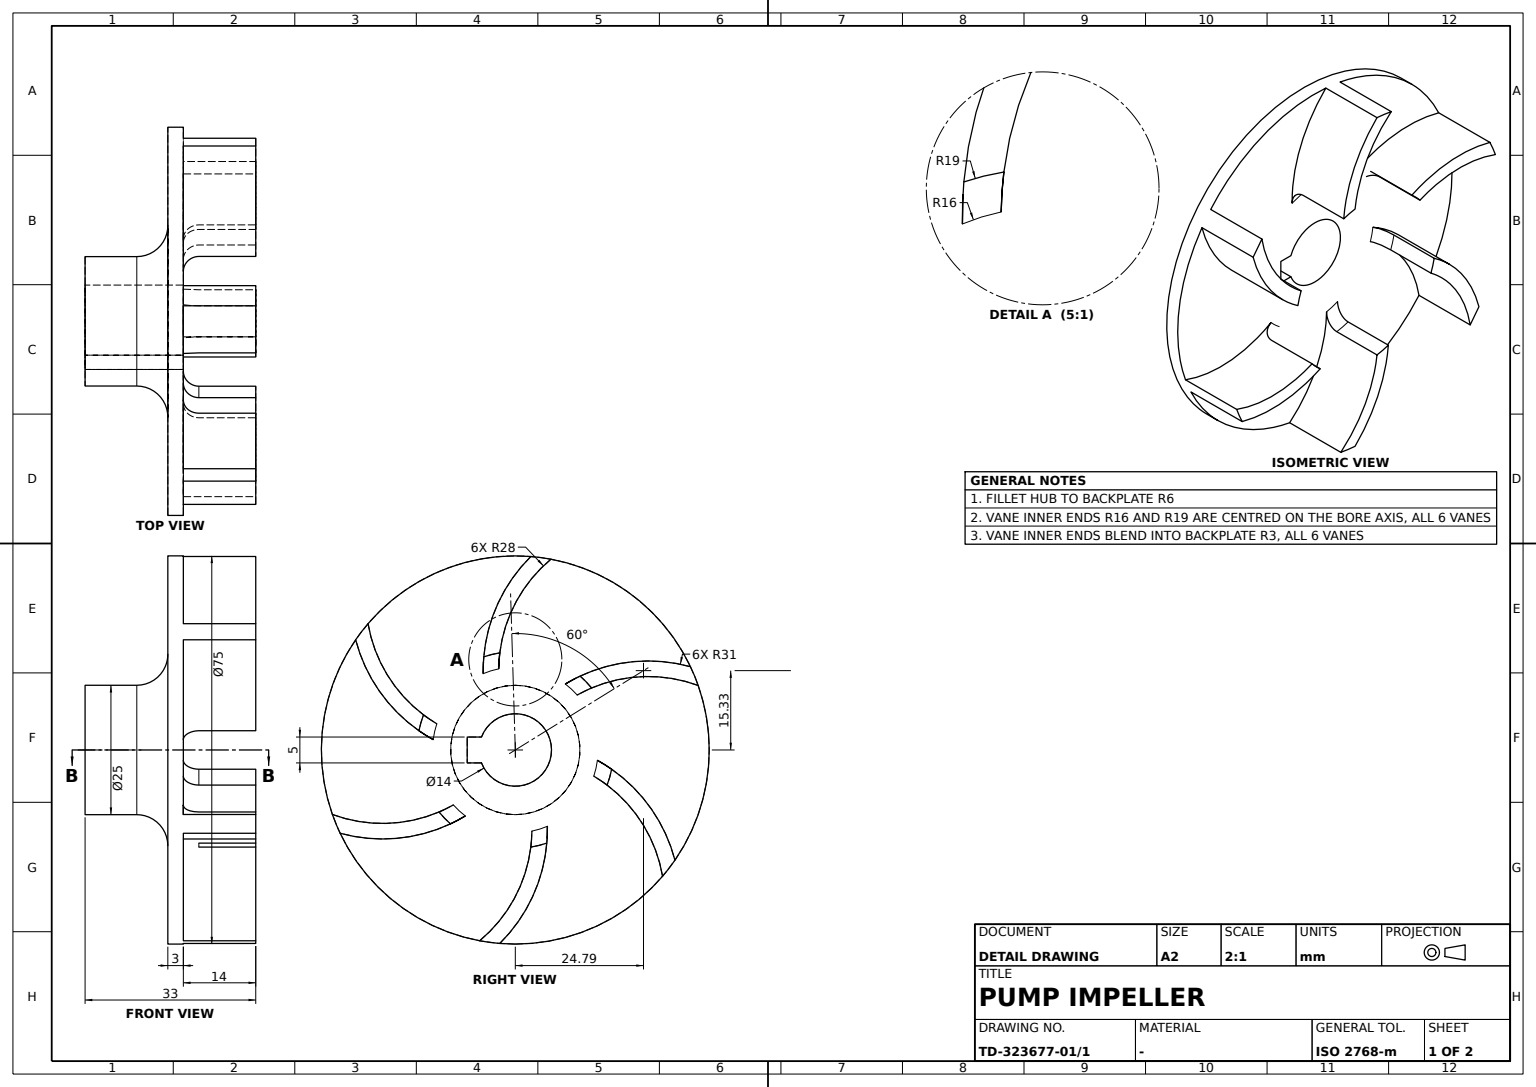
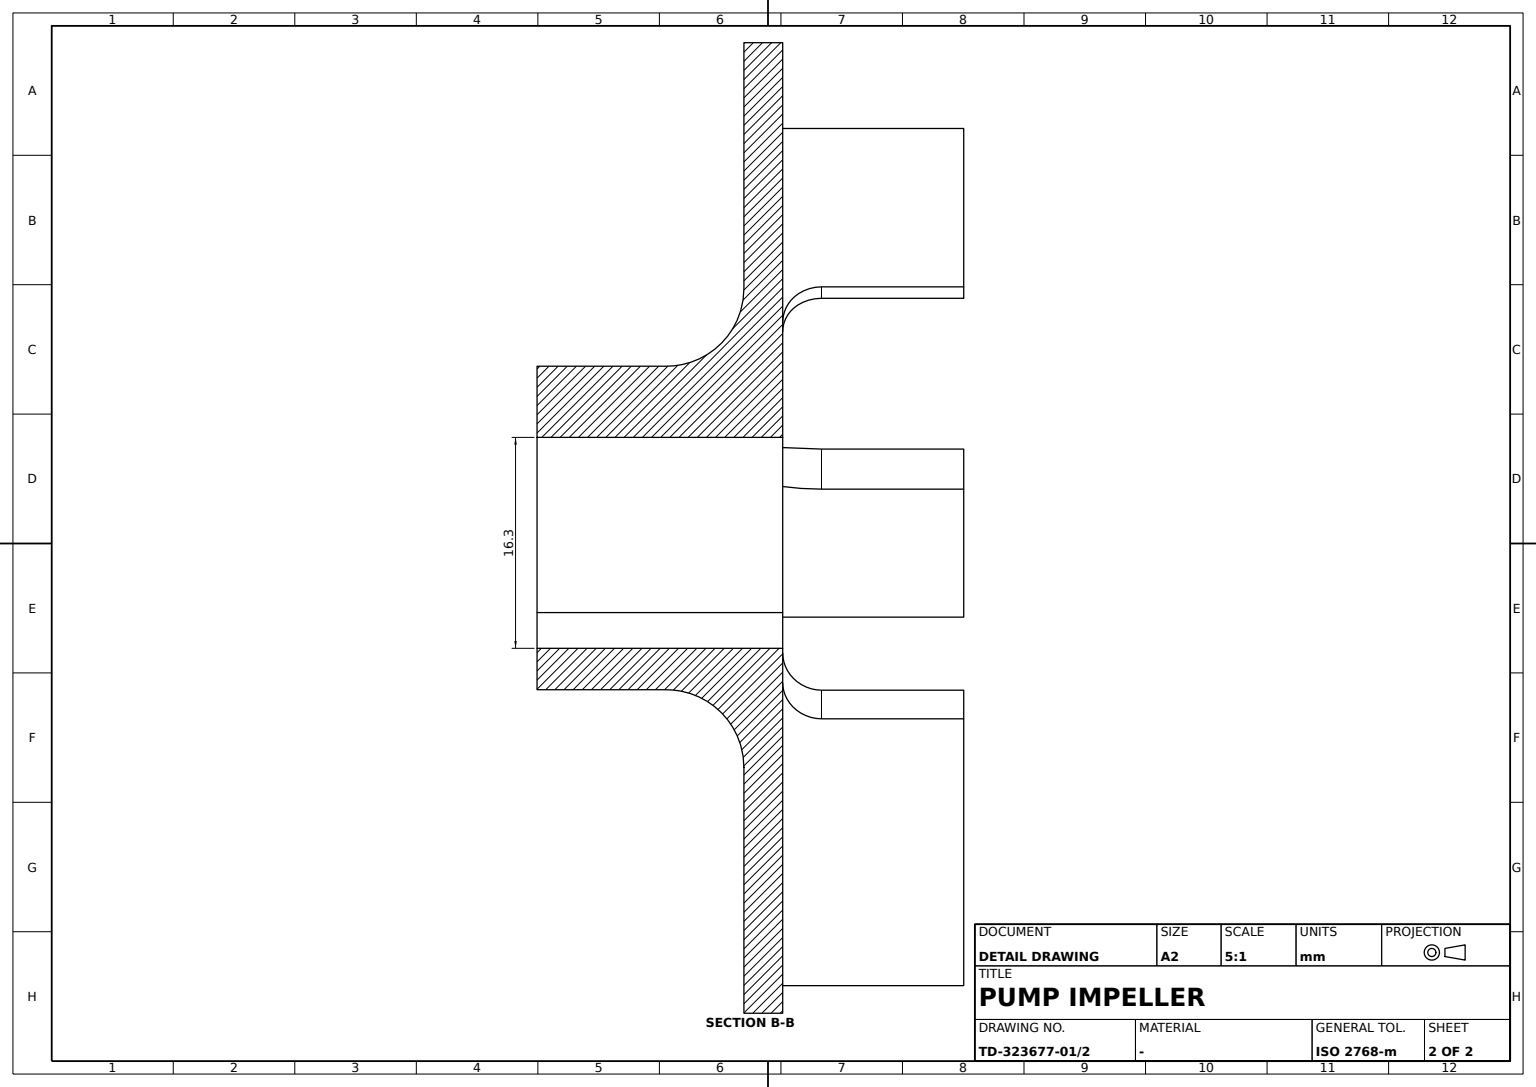
ISO-10303-21;
HEADER;
FILE_DESCRIPTION((''),'2;1');
FILE_NAME('','',(''),(''),'','','');
FILE_SCHEMA(('AUTOMOTIVE_DESIGN'));
ENDSEC;
DATA;
#1=APPLICATION_CONTEXT('');
#2=PRODUCT_CONTEXT('',#1,'mechanical');
#3=PRODUCT('','','',(#2));
#4=PRODUCT_DEFINITION_FORMATION('','',#3);
#5=PRODUCT_DEFINITION_CONTEXT('',#1,'design');
#6=PRODUCT_DEFINITION('','',#4,#5);
#7=PRODUCT_DEFINITION_SHAPE('','',#6);
#8=(LENGTH_UNIT()NAMED_UNIT(*)SI_UNIT(.MILLI.,.METRE.));
#9=(NAMED_UNIT(*)PLANE_ANGLE_UNIT()SI_UNIT($,.RADIAN.));
#10=(NAMED_UNIT(*)SI_UNIT($,.STERADIAN.)SOLID_ANGLE_UNIT());
#11=UNCERTAINTY_MEASURE_WITH_UNIT(LENGTH_MEASURE(0.005),#8,'distance_accuracy_value','');
#12=(GEOMETRIC_REPRESENTATION_CONTEXT(3)GLOBAL_UNCERTAINTY_ASSIGNED_CONTEXT((#11))GLOBAL_UNIT_ASSIGNED_CONTEXT((#8,#9,#10))REPRESENTATION_CONTEXT('',''));
#13=CARTESIAN_POINT('',(-12.5,0.,-16.));
#14=VERTEX_POINT('',#13);
#15=CARTESIAN_POINT('',(0.,0.,-16.));
#16=DIRECTION('',(0.,0.,-1.));
#17=DIRECTION('',(-1.,0.,0.));
#18=AXIS2_PLACEMENT_3D('',#15,#16,#17);
#19=CIRCLE('',#18,12.5);
#20=EDGE_CURVE('',#14,#14,#19,.T.);
#21=ORIENTED_EDGE('',*,*,#20,.F.);
#22=EDGE_LOOP('',(#21));
#23=FACE_BOUND('',#22,.T.);
#24=CARTESIAN_POINT('',(-12.5,0.,-6.));
#25=VERTEX_POINT('',#24);
#26=CARTESIAN_POINT('',(0.,0.,-6.));
#27=AXIS2_PLACEMENT_3D('',#26,#16,#17);
#28=CIRCLE('',#27,12.5);
#29=EDGE_CURVE('',#25,#25,#28,.F.);
#30=ORIENTED_EDGE('',*,*,#29,.F.);
#31=EDGE_LOOP('',(#30));
#32=FACE_BOUND('',#31,.T.);
#33=CARTESIAN_POINT('',(0.,0.,-8.));
#34=DIRECTION('',(1.,0.,0.));
#35=AXIS2_PLACEMENT_3D('',#33,#16,#34);
#36=CYLINDRICAL_SURFACE('',#35,12.5);
#37=ADVANCED_FACE('',(#23,#32),#36,.T.);
#38=CARTESIAN_POINT('',(14.277285,-12.536313,5.999897));
#39=VERTEX_POINT('',#38);
#40=CARTESIAN_POINT('',(14.277285,-12.536313,17.));
#41=VERTEX_POINT('',#40);
#42=DIRECTION('',(0.,0.,1.));
#43=VECTOR('',#42,1000.);
#44=LINE('',#38,#43);
#45=EDGE_CURVE('',#39,#41,#44,.T.);
#46=ORIENTED_EDGE('',*,*,#45,.F.);
#47=CARTESIAN_POINT('',(11.978908,-14.748077,5.9999));
#48=VERTEX_POINT('',#47);
#49=CARTESIAN_POINT('',(0.,0.,6.));
#50=AXIS2_PLACEMENT_3D('',#49,#42,#34);
#51=CIRCLE('',#50,19.);
#52=EDGE_CURVE('',#48,#39,#51,.T.);
#53=ORIENTED_EDGE('',*,*,#52,.F.);
#54=CARTESIAN_POINT('',(11.978908,-14.748077,17.));
#55=VERTEX_POINT('',#54);
#56=LINE('',#47,#43);
#57=EDGE_CURVE('',#48,#55,#56,.T.);
#58=ORIENTED_EDGE('',*,*,#57,.T.);
#59=CARTESIAN_POINT('',(0.,0.,17.));
#60=AXIS2_PLACEMENT_3D('',#59,#42,#34);
#61=CIRCLE('',#60,19.);
#62=EDGE_CURVE('',#55,#41,#61,.T.);
#63=ORIENTED_EDGE('',*,*,#62,.T.);
#64=EDGE_LOOP('',(#46,#53,#58,#63));
#65=FACE_BOUND('',#64,.T.);
#66=CARTESIAN_POINT('',(0.,0.,10.));
#67=DIRECTION('',(0.5,-0.866025404,0.));
#68=AXIS2_PLACEMENT_3D('',#66,#42,#67);
#69=CYLINDRICAL_SURFACE('',#68,19.);
#70=ADVANCED_FACE('',(#65),#69,.F.);
#71=CARTESIAN_POINT('',(-37.379807,3.,17.));
#72=VERTEX_POINT('',#71);
#73=CARTESIAN_POINT('',(-17.995408,-6.096335,17.));
#74=VERTEX_POINT('',#73);
#75=CARTESIAN_POINT('',(-15.328728,24.788756,17.));
#76=AXIS2_PLACEMENT_3D('',#75,#42,#34);
#77=CIRCLE('',#76,31.);
#78=EDGE_CURVE('',#72,#74,#77,.T.);
#79=ORIENTED_EDGE('',*,*,#78,.T.);
#80=CARTESIAN_POINT('',(-18.761663,-3.,17.));
#81=VERTEX_POINT('',#80);
#82=EDGE_CURVE('',#81,#74,#61,.T.);
#83=ORIENTED_EDGE('',*,*,#82,.F.);
#84=CARTESIAN_POINT('',(-36.861476,6.89069,17.));
#85=VERTEX_POINT('',#84);
#86=CIRCLE('',#76,28.);
#87=EDGE_CURVE('',#85,#81,#86,.T.);
#88=ORIENTED_EDGE('',*,*,#87,.F.);
#89=CIRCLE('',#60,37.5);
#90=EDGE_CURVE('',#85,#72,#89,.T.);
#91=ORIENTED_EDGE('',*,*,#90,.T.);
#92=EDGE_LOOP('',(#79,#83,#88,#91));
#93=FACE_BOUND('',#92,.T.);
#94=PLANE('',#60);
#95=ADVANCED_FACE('',(#93),#94,.T.);
#96=CARTESIAN_POINT('',(3.718123,18.632648,5.999897));
#97=VERTEX_POINT('',#96);
#98=CARTESIAN_POINT('',(1.999364,15.874588,3.));
#99=VERTEX_POINT('',#98);
#100=CARTESIAN_POINT('',(3.718106,18.632622,5.173923));
#101=CARTESIAN_POINT('',(3.25884,17.992117,3.591715));
#102=CARTESIAN_POINT('',(2.398072,16.596084,3.));
#103=B_SPLINE_CURVE_WITH_KNOTS('',3,(#96,#100,#101,#102,#98),.UNSPECIFIED.,.F.,.F.,(4,1,4),(0.,0.002441275,0.004882551),.UNSPECIFIED.);
#104=EDGE_CURVE('',#97,#99,#103,.T.);
#105=ORIENTED_EDGE('',*,*,#104,.T.);
#106=CARTESIAN_POINT('',(5.058271,15.179391,3.));
#107=VERTEX_POINT('',#106);
#108=CARTESIAN_POINT('',(0.,0.,3.));
#109=AXIS2_PLACEMENT_3D('',#108,#42,#34);
#110=CIRCLE('',#109,16.);
#111=EDGE_CURVE('',#107,#99,#110,.T.);
#112=ORIENTED_EDGE('',*,*,#111,.F.);
#113=CARTESIAN_POINT('',(6.782755,17.748077,5.9999));
#114=VERTEX_POINT('',#113);
#115=CARTESIAN_POINT('',(6.782738,17.748054,5.195232));
#116=CARTESIAN_POINT('',(6.348912,17.190667,3.633576));
#117=CARTESIAN_POINT('',(5.46887,15.87069,3.));
#118=B_SPLINE_CURVE_WITH_KNOTS('',3,(#113,#115,#116,#117,#106),.UNSPECIFIED.,.F.,.F.,(4,1,4),(0.,0.002379061,0.004758123),.UNSPECIFIED.);
#119=EDGE_CURVE('',#114,#107,#118,.T.);
#120=ORIENTED_EDGE('',*,*,#119,.F.);
#121=EDGE_CURVE('',#114,#97,#51,.T.);
#122=ORIENTED_EDGE('',*,*,#121,.T.);
#123=EDGE_LOOP('',(#105,#112,#120,#122));
#124=FACE_BOUND('',#123,.T.);
#125=DIRECTION('',(0.998937997,-0.046074699,0.));
#126=AXIS2_PLACEMENT_3D('',#49,#42,#125);
#127=TOROIDAL_SURFACE('',#126,16.,3.);
#128=ADVANCED_FACE('',(#124),#127,.F.);
#129=CARTESIAN_POINT('',(-21.28798,-30.871863,17.));
#130=VERTEX_POINT('',#129);
#131=CARTESIAN_POINT('',(-3.718123,-18.632648,17.));
#132=VERTEX_POINT('',#131);
#133=CARTESIAN_POINT('',(-29.132056,-0.88069,17.));
#134=AXIS2_PLACEMENT_3D('',#133,#42,#34);
#135=CIRCLE('',#134,31.);
#136=EDGE_CURVE('',#130,#132,#135,.T.);
#137=ORIENTED_EDGE('',*,*,#136,.T.);
#138=CARTESIAN_POINT('',(-6.782755,-17.748077,17.));
#139=VERTEX_POINT('',#138);
#140=EDGE_CURVE('',#139,#132,#61,.T.);
#141=ORIENTED_EDGE('',*,*,#140,.F.);
#142=CARTESIAN_POINT('',(-24.39825,-28.477629,17.));
#143=VERTEX_POINT('',#142);
#144=CIRCLE('',#134,28.);
#145=EDGE_CURVE('',#143,#139,#144,.T.);
#146=ORIENTED_EDGE('',*,*,#145,.F.);
#147=EDGE_CURVE('',#143,#130,#89,.T.);
#148=ORIENTED_EDGE('',*,*,#147,.T.);
#149=EDGE_LOOP('',(#137,#141,#146,#148));
#150=FACE_BOUND('',#149,.T.);
#151=ADVANCED_FACE('',(#150),#94,.T.);
#152=CARTESIAN_POINT('',(16.091827,-33.871863,3.));
#153=VERTEX_POINT('',#152);
#154=CARTESIAN_POINT('',(12.748115,-9.668794,3.));
#155=VERTEX_POINT('',#154);
#156=CARTESIAN_POINT('',(-13.803329,-25.669446,3.));
#157=AXIS2_PLACEMENT_3D('',#156,#42,#34);
#158=CIRCLE('',#157,31.);
#159=EDGE_CURVE('',#153,#155,#158,.T.);
#160=ORIENTED_EDGE('',*,*,#159,.T.);
#161=CARTESIAN_POINT('',(14.277271,-12.536285,5.173923));
#162=CARTESIAN_POINT('',(13.95221,-11.818297,3.591715));
#163=CARTESIAN_POINT('',(13.173594,-10.374833,3.));
#164=B_SPLINE_CURVE_WITH_KNOTS('',3,(#38,#161,#162,#163,#154),.UNSPECIFIED.,.F.,.F.,(4,1,4),(0.,0.002441275,0.004882551),.UNSPECIFIED.);
#165=EDGE_CURVE('',#39,#155,#164,.T.);
#166=ORIENTED_EDGE('',*,*,#165,.F.);
#167=ORIENTED_EDGE('',*,*,#45,.T.);
#168=CARTESIAN_POINT('',(16.091827,-33.871863,17.));
#169=VERTEX_POINT('',#168);
#170=CARTESIAN_POINT('',(-13.803329,-25.669446,17.));
#171=AXIS2_PLACEMENT_3D('',#170,#42,#34);
#172=CIRCLE('',#171,31.);
#173=EDGE_CURVE('',#169,#41,#172,.T.);
#174=ORIENTED_EDGE('',*,*,#173,.F.);
#175=LINE('',#152,#43);
#176=EDGE_CURVE('',#153,#169,#175,.T.);
#177=ORIENTED_EDGE('',*,*,#176,.F.);
#178=EDGE_LOOP('',(#160,#166,#167,#174,#177));
#179=FACE_BOUND('',#178,.T.);
#180=CARTESIAN_POINT('',(-13.803329,-25.669446,10.));
#181=DIRECTION('',(-0.5,0.866025404,0.));
#182=AXIS2_PLACEMENT_3D('',#180,#42,#181);
#183=CYLINDRICAL_SURFACE('',#182,31.);
#184=ADVANCED_FACE('',(#179),#183,.T.);
#185=CARTESIAN_POINT('',(-18.761663,-3.,5.9999));
#186=VERTEX_POINT('',#185);
#187=LINE('',#185,#43);
#188=EDGE_CURVE('',#186,#81,#187,.T.);
#189=ORIENTED_EDGE('',*,*,#188,.F.);
#190=CARTESIAN_POINT('',(-15.674873,-3.209104,3.));
#191=VERTEX_POINT('',#190);
#192=CARTESIAN_POINT('',(-18.761635,-3.000003,5.195232));
#193=CARTESIAN_POINT('',(-18.06201,-3.097015,3.633576));
#194=CARTESIAN_POINT('',(-16.478856,-3.199165,3.));
#195=B_SPLINE_CURVE_WITH_KNOTS('',3,(#185,#192,#193,#194,#190),.UNSPECIFIED.,.F.,.F.,(4,1,4),(0.,0.002379061,0.004758123),.UNSPECIFIED.);
#196=EDGE_CURVE('',#186,#191,#195,.T.);
#197=ORIENTED_EDGE('',*,*,#196,.T.);
#198=CARTESIAN_POINT('',(-36.861476,6.89069,3.));
#199=VERTEX_POINT('',#198);
#200=CARTESIAN_POINT('',(-15.328728,24.788756,3.));
#201=AXIS2_PLACEMENT_3D('',#200,#42,#34);
#202=CIRCLE('',#201,28.);
#203=EDGE_CURVE('',#199,#191,#202,.T.);
#204=ORIENTED_EDGE('',*,*,#203,.F.);
#205=LINE('',#198,#43);
#206=EDGE_CURVE('',#199,#85,#205,.T.);
#207=ORIENTED_EDGE('',*,*,#206,.T.);
#208=ORIENTED_EDGE('',*,*,#87,.T.);
#209=EDGE_LOOP('',(#189,#197,#204,#207,#208));
#210=FACE_BOUND('',#209,.T.);
#211=CARTESIAN_POINT('',(-15.328728,24.788756,10.));
#212=AXIS2_PLACEMENT_3D('',#211,#42,#34);
#213=CYLINDRICAL_SURFACE('',#212,28.);
#214=ADVANCED_FACE('',(#210),#213,.F.);
#215=ORIENTED_EDGE('',*,*,#20,.T.);
#216=EDGE_LOOP('',(#215));
#217=FACE_BOUND('',#216,.T.);
#218=CARTESIAN_POINT('',(-2.5,-6.538348,-16.));
#219=VERTEX_POINT('',#218);
#220=CARTESIAN_POINT('',(2.5,-6.538348,-16.));
#221=VERTEX_POINT('',#220);
#222=CIRCLE('',#18,7.);
#223=EDGE_CURVE('',#219,#221,#222,.T.);
#224=ORIENTED_EDGE('',*,*,#223,.F.);
#225=CARTESIAN_POINT('',(-2.5,-9.3,-16.));
#226=VERTEX_POINT('',#225);
#227=DIRECTION('',(0.,1.,0.));
#228=VECTOR('',#227,1000.);
#229=LINE('',#225,#228);
#230=EDGE_CURVE('',#226,#219,#229,.T.);
#231=ORIENTED_EDGE('',*,*,#230,.F.);
#232=CARTESIAN_POINT('',(2.5,-9.3,-16.));
#233=VERTEX_POINT('',#232);
#234=VECTOR('',#34,1000.);
#235=LINE('',#225,#234);
#236=EDGE_CURVE('',#226,#233,#235,.T.);
#237=ORIENTED_EDGE('',*,*,#236,.T.);
#238=DIRECTION('',(0.,-1.,0.));
#239=VECTOR('',#238,1000.);
#240=LINE('',#220,#239);
#241=EDGE_CURVE('',#221,#233,#240,.T.);
#242=ORIENTED_EDGE('',*,*,#241,.F.);
#243=EDGE_LOOP('',(#224,#231,#237,#242));
#244=FACE_BOUND('',#243,.T.);
#245=AXIS2_PLACEMENT_3D('',#15,#16,#34);
#246=PLANE('',#245);
#247=ADVANCED_FACE('',(#217,#244),#246,.T.);
#248=ORIENTED_EDGE('',*,*,#119,.T.);
#249=CARTESIAN_POINT('',(24.39825,28.477629,3.));
#250=VERTEX_POINT('',#249);
#251=CARTESIAN_POINT('',(29.132056,0.88069,3.));
#252=AXIS2_PLACEMENT_3D('',#251,#42,#34);
#253=CIRCLE('',#252,28.);
#254=EDGE_CURVE('',#250,#107,#253,.T.);
#255=ORIENTED_EDGE('',*,*,#254,.F.);
#256=CARTESIAN_POINT('',(24.39825,28.477629,17.));
#257=VERTEX_POINT('',#256);
#258=LINE('',#249,#43);
#259=EDGE_CURVE('',#250,#257,#258,.T.);
#260=ORIENTED_EDGE('',*,*,#259,.T.);
#261=CARTESIAN_POINT('',(6.782755,17.748077,17.));
#262=VERTEX_POINT('',#261);
#263=CARTESIAN_POINT('',(29.132056,0.88069,17.));
#264=AXIS2_PLACEMENT_3D('',#263,#42,#34);
#265=CIRCLE('',#264,28.);
#266=EDGE_CURVE('',#257,#262,#265,.T.);
#267=ORIENTED_EDGE('',*,*,#266,.T.);
#268=LINE('',#113,#43);
#269=EDGE_CURVE('',#114,#262,#268,.T.);
#270=ORIENTED_EDGE('',*,*,#269,.F.);
#271=EDGE_LOOP('',(#248,#255,#260,#267,#270));
#272=FACE_BOUND('',#271,.T.);
#273=CARTESIAN_POINT('',(29.132056,0.88069,10.));
#274=DIRECTION('',(-0.5,-0.866025404,0.));
#275=AXIS2_PLACEMENT_3D('',#273,#42,#274);
#276=CYLINDRICAL_SURFACE('',#275,28.);
#277=ADVANCED_FACE('',(#272),#276,.F.);
#278=CARTESIAN_POINT('',(-12.463225,35.368319,17.));
#279=VERTEX_POINT('',#278);
#280=CARTESIAN_POINT('',(-16.091827,33.871863,17.));
#281=VERTEX_POINT('',#280);
#282=EDGE_CURVE('',#279,#281,#89,.T.);
#283=ORIENTED_EDGE('',*,*,#282,.T.);
#284=CARTESIAN_POINT('',(-14.277285,12.536313,17.));
#285=VERTEX_POINT('',#284);
#286=CARTESIAN_POINT('',(13.803329,25.669446,17.));
#287=AXIS2_PLACEMENT_3D('',#286,#42,#34);
#288=CIRCLE('',#287,31.);
#289=EDGE_CURVE('',#281,#285,#288,.T.);
#290=ORIENTED_EDGE('',*,*,#289,.T.);
#291=CARTESIAN_POINT('',(-11.978908,14.748077,17.));
#292=VERTEX_POINT('',#291);
#293=EDGE_CURVE('',#292,#285,#61,.T.);
#294=ORIENTED_EDGE('',*,*,#293,.F.);
#295=CIRCLE('',#287,28.);
#296=EDGE_CURVE('',#279,#292,#295,.T.);
#297=ORIENTED_EDGE('',*,*,#296,.F.);
#298=EDGE_LOOP('',(#283,#290,#294,#297));
#299=FACE_BOUND('',#298,.T.);
#300=ADVANCED_FACE('',(#299),#94,.T.);
#301=CARTESIAN_POINT('',(-17.995408,-6.096335,5.999897));
#302=VERTEX_POINT('',#301);
#303=CARTESIAN_POINT('',(-14.747478,-6.205794,3.));
#304=VERTEX_POINT('',#303);
#305=CARTESIAN_POINT('',(-17.995377,-6.096337,5.173923));
#306=CARTESIAN_POINT('',(-17.211051,-6.17382,3.591715));
#307=CARTESIAN_POINT('',(-15.571666,-6.221251,3.));
#308=B_SPLINE_CURVE_WITH_KNOTS('',3,(#301,#305,#306,#307,#303),.UNSPECIFIED.,.F.,.F.,(4,1,4),(0.,0.002441275,0.004882551),.UNSPECIFIED.);
#309=EDGE_CURVE('',#302,#304,#308,.T.);
#310=ORIENTED_EDGE('',*,*,#309,.F.);
#311=LINE('',#301,#43);
#312=EDGE_CURVE('',#302,#74,#311,.T.);
#313=ORIENTED_EDGE('',*,*,#312,.T.);
#314=ORIENTED_EDGE('',*,*,#78,.F.);
#315=CARTESIAN_POINT('',(-37.379807,3.,3.));
#316=VERTEX_POINT('',#315);
#317=LINE('',#315,#43);
#318=EDGE_CURVE('',#316,#72,#317,.T.);
#319=ORIENTED_EDGE('',*,*,#318,.F.);
#320=CIRCLE('',#201,31.);
#321=EDGE_CURVE('',#316,#304,#320,.T.);
#322=ORIENTED_EDGE('',*,*,#321,.T.);
#323=EDGE_LOOP('',(#310,#313,#314,#319,#322));
#324=FACE_BOUND('',#323,.T.);
#325=CYLINDRICAL_SURFACE('',#212,31.);
#326=ADVANCED_FACE('',(#324),#325,.T.);
#327=ORIENTED_EDGE('',*,*,#165,.T.);
#328=CARTESIAN_POINT('',(10.616603,-11.970286,3.));
#329=VERTEX_POINT('',#328);
#330=EDGE_CURVE('',#329,#155,#110,.T.);
#331=ORIENTED_EDGE('',*,*,#330,.F.);
#332=CARTESIAN_POINT('',(11.978897,-14.748051,5.195232));
#333=CARTESIAN_POINT('',(11.713098,-14.093652,3.633576));
#334=CARTESIAN_POINT('',(11.009986,-12.671526,3.));
#335=B_SPLINE_CURVE_WITH_KNOTS('',3,(#47,#332,#333,#334,#328),.UNSPECIFIED.,.F.,.F.,(4,1,4),(0.,0.002379061,0.004758123),.UNSPECIFIED.);
#336=EDGE_CURVE('',#48,#329,#335,.T.);
#337=ORIENTED_EDGE('',*,*,#336,.F.);
#338=ORIENTED_EDGE('',*,*,#52,.T.);
#339=EDGE_LOOP('',(#327,#331,#337,#338));
#340=FACE_BOUND('',#339,.T.);
#341=ADVANCED_FACE('',(#340),#127,.F.);
#342=CARTESIAN_POINT('',(-3.718123,-18.632648,5.999897));
#343=VERTEX_POINT('',#342);
#344=CARTESIAN_POINT('',(-1.999364,-15.874588,3.));
#345=VERTEX_POINT('',#344);
#346=CARTESIAN_POINT('',(-3.718106,-18.632622,5.173923));
#347=CARTESIAN_POINT('',(-3.25884,-17.992117,3.591715));
#348=CARTESIAN_POINT('',(-2.398072,-16.596084,3.));
#349=B_SPLINE_CURVE_WITH_KNOTS('',3,(#342,#346,#347,#348,#344),.UNSPECIFIED.,.F.,.F.,(4,1,4),(0.,0.002441275,0.004882551),.UNSPECIFIED.);
#350=EDGE_CURVE('',#343,#345,#349,.T.);
#351=ORIENTED_EDGE('',*,*,#350,.T.);
#352=CARTESIAN_POINT('',(-5.058271,-15.179391,3.));
#353=VERTEX_POINT('',#352);
#354=EDGE_CURVE('',#353,#345,#110,.T.);
#355=ORIENTED_EDGE('',*,*,#354,.F.);
#356=CARTESIAN_POINT('',(-6.782755,-17.748077,5.9999));
#357=VERTEX_POINT('',#356);
#358=CARTESIAN_POINT('',(-6.782738,-17.748054,5.195232));
#359=CARTESIAN_POINT('',(-6.348912,-17.190667,3.633576));
#360=CARTESIAN_POINT('',(-5.46887,-15.87069,3.));
#361=B_SPLINE_CURVE_WITH_KNOTS('',3,(#356,#358,#359,#360,#352),.UNSPECIFIED.,.F.,.F.,(4,1,4),(0.,0.002379061,0.004758123),.UNSPECIFIED.);
#362=EDGE_CURVE('',#357,#353,#361,.T.);
#363=ORIENTED_EDGE('',*,*,#362,.F.);
#364=EDGE_CURVE('',#357,#343,#51,.T.);
#365=ORIENTED_EDGE('',*,*,#364,.T.);
#366=EDGE_LOOP('',(#351,#355,#363,#365));
#367=FACE_BOUND('',#366,.T.);
#368=ADVANCED_FACE('',(#367),#127,.F.);
#369=CARTESIAN_POINT('',(-2.5,-9.3,3.));
#370=VERTEX_POINT('',#369);
#371=CARTESIAN_POINT('',(2.5,-9.3,3.));
#372=VERTEX_POINT('',#371);
#373=CARTESIAN_POINT('',(0.,-9.3,3.));
#374=LINE('',#373,#234);
#375=EDGE_CURVE('',#370,#372,#374,.T.);
#376=ORIENTED_EDGE('',*,*,#375,.F.);
#377=CARTESIAN_POINT('',(-2.5,-6.538348,3.));
#378=VERTEX_POINT('',#377);
#379=CARTESIAN_POINT('',(-2.5,0.,3.));
#380=LINE('',#379,#228);
#381=EDGE_CURVE('',#370,#378,#380,.T.);
#382=ORIENTED_EDGE('',*,*,#381,.T.);
#383=CARTESIAN_POINT('',(2.5,-6.538348,3.));
#384=VERTEX_POINT('',#383);
#385=CIRCLE('',#109,7.);
#386=EDGE_CURVE('',#384,#378,#385,.T.);
#387=ORIENTED_EDGE('',*,*,#386,.F.);
#388=CARTESIAN_POINT('',(2.5,0.,3.));
#389=LINE('',#388,#239);
#390=EDGE_CURVE('',#384,#372,#389,.T.);
#391=ORIENTED_EDGE('',*,*,#390,.T.);
#392=EDGE_LOOP('',(#376,#382,#387,#391));
#393=FACE_BOUND('',#392,.T.);
#394=CARTESIAN_POINT('',(-12.463225,35.368319,3.));
#395=VERTEX_POINT('',#394);
#396=CARTESIAN_POINT('',(-10.616603,11.970286,3.));
#397=VERTEX_POINT('',#396);
#398=CARTESIAN_POINT('',(13.803329,25.669446,3.));
#399=AXIS2_PLACEMENT_3D('',#398,#42,#34);
#400=CIRCLE('',#399,28.);
#401=EDGE_CURVE('',#395,#397,#400,.T.);
#402=ORIENTED_EDGE('',*,*,#401,.T.);
#403=CARTESIAN_POINT('',(-12.748115,9.668794,3.));
#404=VERTEX_POINT('',#403);
#405=EDGE_CURVE('',#397,#404,#110,.T.);
#406=ORIENTED_EDGE('',*,*,#405,.T.);
#407=CARTESIAN_POINT('',(-16.091827,33.871863,3.));
#408=VERTEX_POINT('',#407);
#409=CIRCLE('',#399,31.);
#410=EDGE_CURVE('',#408,#404,#409,.T.);
#411=ORIENTED_EDGE('',*,*,#410,.F.);
#412=CIRCLE('',#109,37.5);
#413=EDGE_CURVE('',#408,#199,#412,.T.);
#414=ORIENTED_EDGE('',*,*,#413,.T.);
#415=ORIENTED_EDGE('',*,*,#203,.T.);
#416=EDGE_CURVE('',#191,#304,#110,.T.);
#417=ORIENTED_EDGE('',*,*,#416,.T.);
#418=ORIENTED_EDGE('',*,*,#321,.F.);
#419=CARTESIAN_POINT('',(-24.39825,-28.477629,3.));
#420=VERTEX_POINT('',#419);
#421=EDGE_CURVE('',#316,#420,#412,.T.);
#422=ORIENTED_EDGE('',*,*,#421,.T.);
#423=CARTESIAN_POINT('',(-29.132056,-0.88069,3.));
#424=AXIS2_PLACEMENT_3D('',#423,#42,#34);
#425=CIRCLE('',#424,28.);
#426=EDGE_CURVE('',#420,#353,#425,.T.);
#427=ORIENTED_EDGE('',*,*,#426,.T.);
#428=ORIENTED_EDGE('',*,*,#354,.T.);
#429=CARTESIAN_POINT('',(-21.28798,-30.871863,3.));
#430=VERTEX_POINT('',#429);
#431=CIRCLE('',#424,31.);
#432=EDGE_CURVE('',#430,#345,#431,.T.);
#433=ORIENTED_EDGE('',*,*,#432,.F.);
#434=CARTESIAN_POINT('',(12.463225,-35.368319,3.));
#435=VERTEX_POINT('',#434);
#436=EDGE_CURVE('',#430,#435,#412,.T.);
#437=ORIENTED_EDGE('',*,*,#436,.T.);
#438=CIRCLE('',#157,28.);
#439=EDGE_CURVE('',#435,#329,#438,.T.);
#440=ORIENTED_EDGE('',*,*,#439,.T.);
#441=ORIENTED_EDGE('',*,*,#330,.T.);
#442=ORIENTED_EDGE('',*,*,#159,.F.);
#443=CARTESIAN_POINT('',(36.861476,-6.89069,3.));
#444=VERTEX_POINT('',#443);
#445=EDGE_CURVE('',#153,#444,#412,.T.);
#446=ORIENTED_EDGE('',*,*,#445,.T.);
#447=CARTESIAN_POINT('',(15.674873,3.209104,3.));
#448=VERTEX_POINT('',#447);
#449=CARTESIAN_POINT('',(15.328728,-24.788756,3.));
#450=AXIS2_PLACEMENT_3D('',#449,#42,#34);
#451=CIRCLE('',#450,28.);
#452=EDGE_CURVE('',#444,#448,#451,.T.);
#453=ORIENTED_EDGE('',*,*,#452,.T.);
#454=CARTESIAN_POINT('',(14.747478,6.205794,3.));
#455=VERTEX_POINT('',#454);
#456=EDGE_CURVE('',#448,#455,#110,.T.);
#457=ORIENTED_EDGE('',*,*,#456,.T.);
#458=CARTESIAN_POINT('',(37.379807,-3.,3.));
#459=VERTEX_POINT('',#458);
#460=CIRCLE('',#450,31.);
#461=EDGE_CURVE('',#459,#455,#460,.T.);
#462=ORIENTED_EDGE('',*,*,#461,.F.);
#463=EDGE_CURVE('',#459,#250,#412,.T.);
#464=ORIENTED_EDGE('',*,*,#463,.T.);
#465=ORIENTED_EDGE('',*,*,#254,.T.);
#466=ORIENTED_EDGE('',*,*,#111,.T.);
#467=CARTESIAN_POINT('',(21.28798,30.871863,3.));
#468=VERTEX_POINT('',#467);
#469=CIRCLE('',#252,31.);
#470=EDGE_CURVE('',#468,#99,#469,.T.);
#471=ORIENTED_EDGE('',*,*,#470,.F.);
#472=EDGE_CURVE('',#468,#395,#412,.T.);
#473=ORIENTED_EDGE('',*,*,#472,.T.);
#474=EDGE_LOOP('',(#402,#406,#411,#414,#415,#417,#418,#422,#427,#428,#433,#437,#440,#441,#442,#446,#453,#457,#462,#464,#465,#466,#471,#473));
#475=FACE_BOUND('',#474,.T.);
#476=PLANE('',#109);
#477=ADVANCED_FACE('',(#393,#475),#476,.T.);
#478=CARTESIAN_POINT('',(17.995408,6.096335,5.999897));
#479=VERTEX_POINT('',#478);
#480=CARTESIAN_POINT('',(17.995377,6.096337,5.173923));
#481=CARTESIAN_POINT('',(17.211051,6.17382,3.591715));
#482=CARTESIAN_POINT('',(15.571666,6.221251,3.));
#483=B_SPLINE_CURVE_WITH_KNOTS('',3,(#478,#480,#481,#482,#454),.UNSPECIFIED.,.F.,.F.,(4,1,4),(0.,0.002441275,0.004882551),.UNSPECIFIED.);
#484=EDGE_CURVE('',#479,#455,#483,.T.);
#485=ORIENTED_EDGE('',*,*,#484,.T.);
#486=ORIENTED_EDGE('',*,*,#456,.F.);
#487=CARTESIAN_POINT('',(18.761663,3.,5.9999));
#488=VERTEX_POINT('',#487);
#489=CARTESIAN_POINT('',(18.761635,3.000003,5.195232));
#490=CARTESIAN_POINT('',(18.06201,3.097015,3.633576));
#491=CARTESIAN_POINT('',(16.478856,3.199165,3.));
#492=B_SPLINE_CURVE_WITH_KNOTS('',3,(#487,#489,#490,#491,#447),.UNSPECIFIED.,.F.,.F.,(4,1,4),(0.,0.002379061,0.004758123),.UNSPECIFIED.);
#493=EDGE_CURVE('',#488,#448,#492,.T.);
#494=ORIENTED_EDGE('',*,*,#493,.F.);
#495=EDGE_CURVE('',#488,#479,#51,.T.);
#496=ORIENTED_EDGE('',*,*,#495,.T.);
#497=EDGE_LOOP('',(#485,#486,#494,#496));
#498=FACE_BOUND('',#497,.T.);
#499=ADVANCED_FACE('',(#498),#127,.F.);
#500=CARTESIAN_POINT('',(36.861476,-6.89069,17.));
#501=VERTEX_POINT('',#500);
#502=LINE('',#443,#43);
#503=EDGE_CURVE('',#444,#501,#502,.T.);
#504=ORIENTED_EDGE('',*,*,#503,.T.);
#505=CARTESIAN_POINT('',(18.761663,3.,17.));
#506=VERTEX_POINT('',#505);
#507=CARTESIAN_POINT('',(15.328728,-24.788756,17.));
#508=AXIS2_PLACEMENT_3D('',#507,#42,#34);
#509=CIRCLE('',#508,28.);
#510=EDGE_CURVE('',#501,#506,#509,.T.);
#511=ORIENTED_EDGE('',*,*,#510,.T.);
#512=LINE('',#487,#43);
#513=EDGE_CURVE('',#488,#506,#512,.T.);
#514=ORIENTED_EDGE('',*,*,#513,.F.);
#515=ORIENTED_EDGE('',*,*,#493,.T.);
#516=ORIENTED_EDGE('',*,*,#452,.F.);
#517=EDGE_LOOP('',(#504,#511,#514,#515,#516));
#518=FACE_BOUND('',#517,.T.);
#519=CARTESIAN_POINT('',(15.328728,-24.788756,10.));
#520=AXIS2_PLACEMENT_3D('',#519,#42,#17);
#521=CYLINDRICAL_SURFACE('',#520,28.);
#522=ADVANCED_FACE('',(#518),#521,.F.);
#523=LINE('',#356,#43);
#524=EDGE_CURVE('',#357,#139,#523,.T.);
#525=ORIENTED_EDGE('',*,*,#524,.T.);
#526=ORIENTED_EDGE('',*,*,#140,.T.);
#527=LINE('',#342,#43);
#528=EDGE_CURVE('',#343,#132,#527,.T.);
#529=ORIENTED_EDGE('',*,*,#528,.F.);
#530=ORIENTED_EDGE('',*,*,#364,.F.);
#531=EDGE_LOOP('',(#525,#526,#529,#530));
#532=FACE_BOUND('',#531,.T.);
#533=ADVANCED_FACE('',(#532),#69,.F.);
#534=CARTESIAN_POINT('',(3.718123,18.632648,17.));
#535=VERTEX_POINT('',#534);
#536=LINE('',#96,#43);
#537=EDGE_CURVE('',#97,#535,#536,.T.);
#538=ORIENTED_EDGE('',*,*,#537,.F.);
#539=ORIENTED_EDGE('',*,*,#121,.F.);
#540=ORIENTED_EDGE('',*,*,#269,.T.);
#541=EDGE_CURVE('',#262,#535,#61,.T.);
#542=ORIENTED_EDGE('',*,*,#541,.T.);
#543=EDGE_LOOP('',(#538,#539,#540,#542));
#544=FACE_BOUND('',#543,.T.);
#545=ADVANCED_FACE('',(#544),#69,.F.);
#546=CARTESIAN_POINT('',(17.995408,6.096335,17.));
#547=VERTEX_POINT('',#546);
#548=LINE('',#478,#43);
#549=EDGE_CURVE('',#479,#547,#548,.T.);
#550=ORIENTED_EDGE('',*,*,#549,.T.);
#551=CARTESIAN_POINT('',(37.379807,-3.,17.));
#552=VERTEX_POINT('',#551);
#553=CIRCLE('',#508,31.);
#554=EDGE_CURVE('',#552,#547,#553,.T.);
#555=ORIENTED_EDGE('',*,*,#554,.F.);
#556=LINE('',#458,#43);
#557=EDGE_CURVE('',#459,#552,#556,.T.);
#558=ORIENTED_EDGE('',*,*,#557,.F.);
#559=ORIENTED_EDGE('',*,*,#461,.T.);
#560=ORIENTED_EDGE('',*,*,#484,.F.);
#561=EDGE_LOOP('',(#550,#555,#558,#559,#560));
#562=FACE_BOUND('',#561,.T.);
#563=CYLINDRICAL_SURFACE('',#520,31.);
#564=ADVANCED_FACE('',(#562),#563,.T.);
#565=CARTESIAN_POINT('',(37.5,0.,0.));
#566=VERTEX_POINT('',#565);
#567=CARTESIAN_POINT('',(0.,0.,0.));
#568=AXIS2_PLACEMENT_3D('',#567,#42,#34);
#569=CIRCLE('',#568,37.5);
#570=EDGE_CURVE('',#566,#566,#569,.T.);
#571=ORIENTED_EDGE('',*,*,#570,.F.);
#572=EDGE_LOOP('',(#571));
#573=FACE_BOUND('',#572,.T.);
#574=CARTESIAN_POINT('',(18.5,0.,0.));
#575=VERTEX_POINT('',#574);
#576=CIRCLE('',#568,18.5);
#577=EDGE_CURVE('',#575,#575,#576,.T.);
#578=ORIENTED_EDGE('',*,*,#577,.T.);
#579=EDGE_LOOP('',(#578));
#580=FACE_BOUND('',#579,.T.);
#581=PLANE('',#568);
#582=ADVANCED_FACE('',(#573,#580),#581,.F.);
#583=ORIENTED_EDGE('',*,*,#173,.T.);
#584=ORIENTED_EDGE('',*,*,#62,.F.);
#585=CARTESIAN_POINT('',(12.463225,-35.368319,17.));
#586=VERTEX_POINT('',#585);
#587=CIRCLE('',#171,28.);
#588=EDGE_CURVE('',#586,#55,#587,.T.);
#589=ORIENTED_EDGE('',*,*,#588,.F.);
#590=EDGE_CURVE('',#586,#169,#89,.T.);
#591=ORIENTED_EDGE('',*,*,#590,.T.);
#592=EDGE_LOOP('',(#583,#584,#589,#591));
#593=FACE_BOUND('',#592,.T.);
#594=ADVANCED_FACE('',(#593),#94,.T.);
#595=ORIENTED_EDGE('',*,*,#570,.T.);
#596=EDGE_LOOP('',(#595));
#597=FACE_BOUND('',#596,.T.);
#598=ORIENTED_EDGE('',*,*,#436,.F.);
#599=LINE('',#429,#43);
#600=EDGE_CURVE('',#430,#130,#599,.T.);
#601=ORIENTED_EDGE('',*,*,#600,.T.);
#602=ORIENTED_EDGE('',*,*,#147,.F.);
#603=LINE('',#419,#43);
#604=EDGE_CURVE('',#420,#143,#603,.T.);
#605=ORIENTED_EDGE('',*,*,#604,.F.);
#606=ORIENTED_EDGE('',*,*,#421,.F.);
#607=ORIENTED_EDGE('',*,*,#318,.T.);
#608=ORIENTED_EDGE('',*,*,#90,.F.);
#609=ORIENTED_EDGE('',*,*,#206,.F.);
#610=ORIENTED_EDGE('',*,*,#413,.F.);
#611=LINE('',#407,#43);
#612=EDGE_CURVE('',#408,#281,#611,.T.);
#613=ORIENTED_EDGE('',*,*,#612,.T.);
#614=ORIENTED_EDGE('',*,*,#282,.F.);
#615=LINE('',#394,#43);
#616=EDGE_CURVE('',#395,#279,#615,.T.);
#617=ORIENTED_EDGE('',*,*,#616,.F.);
#618=ORIENTED_EDGE('',*,*,#472,.F.);
#619=CARTESIAN_POINT('',(21.28798,30.871863,17.));
#620=VERTEX_POINT('',#619);
#621=LINE('',#467,#43);
#622=EDGE_CURVE('',#468,#620,#621,.T.);
#623=ORIENTED_EDGE('',*,*,#622,.T.);
#624=EDGE_CURVE('',#257,#620,#89,.T.);
#625=ORIENTED_EDGE('',*,*,#624,.F.);
#626=ORIENTED_EDGE('',*,*,#259,.F.);
#627=ORIENTED_EDGE('',*,*,#463,.F.);
#628=ORIENTED_EDGE('',*,*,#557,.T.);
#629=EDGE_CURVE('',#501,#552,#89,.T.);
#630=ORIENTED_EDGE('',*,*,#629,.F.);
#631=ORIENTED_EDGE('',*,*,#503,.F.);
#632=ORIENTED_EDGE('',*,*,#445,.F.);
#633=ORIENTED_EDGE('',*,*,#176,.T.);
#634=ORIENTED_EDGE('',*,*,#590,.F.);
#635=LINE('',#434,#43);
#636=EDGE_CURVE('',#435,#586,#635,.T.);
#637=ORIENTED_EDGE('',*,*,#636,.F.);
#638=EDGE_LOOP('',(#598,#601,#602,#605,#606,#607,#608,#609,#610,#613,#614,#617,#618,#623,#625,#626,#627,#628,#630,#631,#632,#633,#634,#637));
#639=FACE_BOUND('',#638,.T.);
#640=CARTESIAN_POINT('',(0.,0.,1.5));
#641=AXIS2_PLACEMENT_3D('',#640,#42,#34);
#642=CYLINDRICAL_SURFACE('',#641,37.5);
#643=ADVANCED_FACE('',(#597,#639),#642,.T.);
#644=CARTESIAN_POINT('',(-11.978908,14.748077,6.));
#645=VERTEX_POINT('',#644);
#646=LINE('',#644,#43);
#647=EDGE_CURVE('',#645,#292,#646,.T.);
#648=ORIENTED_EDGE('',*,*,#647,.T.);
#649=ORIENTED_EDGE('',*,*,#293,.T.);
#650=CARTESIAN_POINT('',(-14.277285,12.536313,6.));
#651=VERTEX_POINT('',#650);
#652=LINE('',#650,#43);
#653=EDGE_CURVE('',#651,#285,#652,.T.);
#654=ORIENTED_EDGE('',*,*,#653,.F.);
#655=EDGE_CURVE('',#645,#651,#51,.T.);
#656=ORIENTED_EDGE('',*,*,#655,.F.);
#657=EDGE_LOOP('',(#648,#649,#654,#656));
#658=FACE_BOUND('',#657,.T.);
#659=ADVANCED_FACE('',(#658),#69,.F.);
#660=ORIENTED_EDGE('',*,*,#549,.F.);
#661=ORIENTED_EDGE('',*,*,#495,.F.);
#662=ORIENTED_EDGE('',*,*,#513,.T.);
#663=EDGE_CURVE('',#506,#547,#61,.T.);
#664=ORIENTED_EDGE('',*,*,#663,.T.);
#665=EDGE_LOOP('',(#660,#661,#662,#664));
#666=FACE_BOUND('',#665,.T.);
#667=ADVANCED_FACE('',(#666),#69,.F.);
#668=ORIENTED_EDGE('',*,*,#241,.T.);
#669=LINE('',#232,#43);
#670=EDGE_CURVE('',#233,#372,#669,.T.);
#671=ORIENTED_EDGE('',*,*,#670,.T.);
#672=ORIENTED_EDGE('',*,*,#390,.F.);
#673=VECTOR('',#16,1000.);
#674=LINE('',#220,#673);
#675=EDGE_CURVE('',#221,#384,#674,.F.);
#676=ORIENTED_EDGE('',*,*,#675,.F.);
#677=EDGE_LOOP('',(#668,#671,#672,#676));
#678=FACE_BOUND('',#677,.T.);
#679=AXIS2_PLACEMENT_3D('',#220,#17,#238);
#680=PLANE('',#679);
#681=ADVANCED_FACE('',(#678),#680,.T.);
#682=ORIENTED_EDGE('',*,*,#375,.T.);
#683=ORIENTED_EDGE('',*,*,#670,.F.);
#684=ORIENTED_EDGE('',*,*,#236,.F.);
#685=LINE('',#225,#43);
#686=EDGE_CURVE('',#226,#370,#685,.T.);
#687=ORIENTED_EDGE('',*,*,#686,.T.);
#688=EDGE_LOOP('',(#682,#683,#684,#687));
#689=FACE_BOUND('',#688,.T.);
#690=AXIS2_PLACEMENT_3D('',#225,#238,#34);
#691=PLANE('',#690);
#692=ADVANCED_FACE('',(#689),#691,.F.);
#693=ORIENTED_EDGE('',*,*,#309,.T.);
#694=ORIENTED_EDGE('',*,*,#416,.F.);
#695=ORIENTED_EDGE('',*,*,#196,.F.);
#696=EDGE_CURVE('',#186,#302,#51,.T.);
#697=ORIENTED_EDGE('',*,*,#696,.T.);
#698=EDGE_LOOP('',(#693,#694,#695,#697));
#699=FACE_BOUND('',#698,.T.);
#700=ADVANCED_FACE('',(#699),#127,.F.);
#701=LINE('',#218,#673);
#702=EDGE_CURVE('',#219,#378,#701,.F.);
#703=ORIENTED_EDGE('',*,*,#702,.T.);
#704=ORIENTED_EDGE('',*,*,#381,.F.);
#705=ORIENTED_EDGE('',*,*,#686,.F.);
#706=ORIENTED_EDGE('',*,*,#230,.T.);
#707=EDGE_LOOP('',(#703,#704,#705,#706));
#708=FACE_BOUND('',#707,.T.);
#709=AXIS2_PLACEMENT_3D('',#225,#34,#227);
#710=PLANE('',#709);
#711=ADVANCED_FACE('',(#708),#710,.T.);
#712=ORIENTED_EDGE('',*,*,#336,.T.);
#713=ORIENTED_EDGE('',*,*,#439,.F.);
#714=ORIENTED_EDGE('',*,*,#636,.T.);
#715=ORIENTED_EDGE('',*,*,#588,.T.);
#716=ORIENTED_EDGE('',*,*,#57,.F.);
#717=EDGE_LOOP('',(#712,#713,#714,#715,#716));
#718=FACE_BOUND('',#717,.T.);
#719=CYLINDRICAL_SURFACE('',#182,28.);
#720=ADVANCED_FACE('',(#718),#719,.F.);
#721=ORIENTED_EDGE('',*,*,#266,.F.);
#722=ORIENTED_EDGE('',*,*,#624,.T.);
#723=CIRCLE('',#264,31.);
#724=EDGE_CURVE('',#620,#535,#723,.T.);
#725=ORIENTED_EDGE('',*,*,#724,.T.);
#726=ORIENTED_EDGE('',*,*,#541,.F.);
#727=EDGE_LOOP('',(#721,#722,#725,#726));
#728=FACE_BOUND('',#727,.T.);
#729=ADVANCED_FACE('',(#728),#94,.T.);
#730=ORIENTED_EDGE('',*,*,#312,.F.);
#731=ORIENTED_EDGE('',*,*,#696,.F.);
#732=ORIENTED_EDGE('',*,*,#188,.T.);
#733=ORIENTED_EDGE('',*,*,#82,.T.);
#734=EDGE_LOOP('',(#730,#731,#732,#733));
#735=FACE_BOUND('',#734,.T.);
#736=ADVANCED_FACE('',(#735),#69,.F.);
#737=CARTESIAN_POINT('',(-11.978908,14.748077,5.195315));
#738=CARTESIAN_POINT('',(-11.713119,14.093697,3.633604));
#739=CARTESIAN_POINT('',(-11.009994,12.671541,3.));
#740=B_SPLINE_CURVE_WITH_KNOTS('',3,(#644,#737,#738,#739,#396),.UNSPECIFIED.,.F.,.F.,(4,1,4),(0.,0.002379112,0.004758223),.UNSPECIFIED.);
#741=EDGE_CURVE('',#645,#397,#740,.T.);
#742=ORIENTED_EDGE('',*,*,#741,.T.);
#743=ORIENTED_EDGE('',*,*,#401,.F.);
#744=ORIENTED_EDGE('',*,*,#616,.T.);
#745=ORIENTED_EDGE('',*,*,#296,.T.);
#746=ORIENTED_EDGE('',*,*,#647,.F.);
#747=EDGE_LOOP('',(#742,#743,#744,#745,#746));
#748=FACE_BOUND('',#747,.T.);
#749=CARTESIAN_POINT('',(13.803329,25.669446,10.));
#750=AXIS2_PLACEMENT_3D('',#749,#42,#67);
#751=CYLINDRICAL_SURFACE('',#750,28.);
#752=ADVANCED_FACE('',(#748),#751,.F.);
#753=ORIENTED_EDGE('',*,*,#470,.T.);
#754=ORIENTED_EDGE('',*,*,#104,.F.);
#755=ORIENTED_EDGE('',*,*,#537,.T.);
#756=ORIENTED_EDGE('',*,*,#724,.F.);
#757=ORIENTED_EDGE('',*,*,#622,.F.);
#758=EDGE_LOOP('',(#753,#754,#755,#756,#757));
#759=FACE_BOUND('',#758,.T.);
#760=CYLINDRICAL_SURFACE('',#275,31.);
#761=ADVANCED_FACE('',(#759),#760,.T.);
#762=ORIENTED_EDGE('',*,*,#655,.T.);
#763=CARTESIAN_POINT('',(-14.277285,12.536313,5.174009));
#764=CARTESIAN_POINT('',(-13.952234,11.818344,3.59174));
#765=CARTESIAN_POINT('',(-13.173603,10.374848,3.));
#766=B_SPLINE_CURVE_WITH_KNOTS('',3,(#650,#763,#764,#765,#403),.UNSPECIFIED.,.F.,.F.,(4,1,4),(0.,0.002441327,0.004882655),.UNSPECIFIED.);
#767=EDGE_CURVE('',#651,#404,#766,.T.);
#768=ORIENTED_EDGE('',*,*,#767,.T.);
#769=ORIENTED_EDGE('',*,*,#405,.F.);
#770=ORIENTED_EDGE('',*,*,#741,.F.);
#771=EDGE_LOOP('',(#762,#768,#769,#770));
#772=FACE_BOUND('',#771,.T.);
#773=ADVANCED_FACE('',(#772),#127,.F.);
#774=ORIENTED_EDGE('',*,*,#604,.T.);
#775=ORIENTED_EDGE('',*,*,#145,.T.);
#776=ORIENTED_EDGE('',*,*,#524,.F.);
#777=ORIENTED_EDGE('',*,*,#362,.T.);
#778=ORIENTED_EDGE('',*,*,#426,.F.);
#779=EDGE_LOOP('',(#774,#775,#776,#777,#778));
#780=FACE_BOUND('',#779,.T.);
#781=CARTESIAN_POINT('',(-29.132056,-0.88069,10.));
#782=DIRECTION('',(0.5,0.866025404,0.));
#783=AXIS2_PLACEMENT_3D('',#781,#42,#782);
#784=CYLINDRICAL_SURFACE('',#783,28.);
#785=ADVANCED_FACE('',(#780),#784,.F.);
#786=ORIENTED_EDGE('',*,*,#289,.F.);
#787=ORIENTED_EDGE('',*,*,#612,.F.);
#788=ORIENTED_EDGE('',*,*,#410,.T.);
#789=ORIENTED_EDGE('',*,*,#767,.F.);
#790=ORIENTED_EDGE('',*,*,#653,.T.);
#791=EDGE_LOOP('',(#786,#787,#788,#789,#790));
#792=FACE_BOUND('',#791,.T.);
#793=CYLINDRICAL_SURFACE('',#750,31.);
#794=ADVANCED_FACE('',(#792),#793,.T.);
#795=ORIENTED_EDGE('',*,*,#577,.F.);
#796=EDGE_LOOP('',(#795));
#797=FACE_BOUND('',#796,.T.);
#798=ORIENTED_EDGE('',*,*,#29,.T.);
#799=EDGE_LOOP('',(#798));
#800=FACE_BOUND('',#799,.T.);
#801=DIRECTION('',(0.744123466,-0.668042115,0.));
#802=AXIS2_PLACEMENT_3D('',#26,#42,#801);
#803=TOROIDAL_SURFACE('',#802,18.5,6.);
#804=ADVANCED_FACE('',(#797,#800),#803,.F.);
#805=ORIENTED_EDGE('',*,*,#528,.T.);
#806=ORIENTED_EDGE('',*,*,#136,.F.);
#807=ORIENTED_EDGE('',*,*,#600,.F.);
#808=ORIENTED_EDGE('',*,*,#432,.T.);
#809=ORIENTED_EDGE('',*,*,#350,.F.);
#810=EDGE_LOOP('',(#805,#806,#807,#808,#809));
#811=FACE_BOUND('',#810,.T.);
#812=CYLINDRICAL_SURFACE('',#783,31.);
#813=ADVANCED_FACE('',(#811),#812,.T.);
#814=ORIENTED_EDGE('',*,*,#223,.T.);
#815=ORIENTED_EDGE('',*,*,#675,.T.);
#816=ORIENTED_EDGE('',*,*,#386,.T.);
#817=ORIENTED_EDGE('',*,*,#702,.F.);
#818=EDGE_LOOP('',(#814,#815,#816,#817));
#819=FACE_BOUND('',#818,.T.);
#820=CARTESIAN_POINT('',(0.,0.,9.5));
#821=AXIS2_PLACEMENT_3D('',#820,#16,#34);
#822=CYLINDRICAL_SURFACE('',#821,7.);
#823=ADVANCED_FACE('',(#819),#822,.F.);
#824=ORIENTED_EDGE('',*,*,#554,.T.);
#825=ORIENTED_EDGE('',*,*,#663,.F.);
#826=ORIENTED_EDGE('',*,*,#510,.F.);
#827=ORIENTED_EDGE('',*,*,#629,.T.);
#828=EDGE_LOOP('',(#824,#825,#826,#827));
#829=FACE_BOUND('',#828,.T.);
#830=ADVANCED_FACE('',(#829),#94,.T.);
#831=CLOSED_SHELL('',(#37,#70,#95,#128,#151,#184,#214,#247,#277,#300,#326,#341,#368,#477,#499,#522,#533,#545,#564,#582,#594,#643,#659,#667,#681,#692,#700,#711,#720,#729,#736,#752,#761,#773,#785,#794,#804,#813,#823,#830));
#832=MANIFOLD_SOLID_BREP('',#831);
#833=ADVANCED_BREP_SHAPE_REPRESENTATION('',(#832),#12);
#834=SHAPE_DEFINITION_REPRESENTATION(#7,#833);
ENDSEC;
END-ISO-10303-21;
